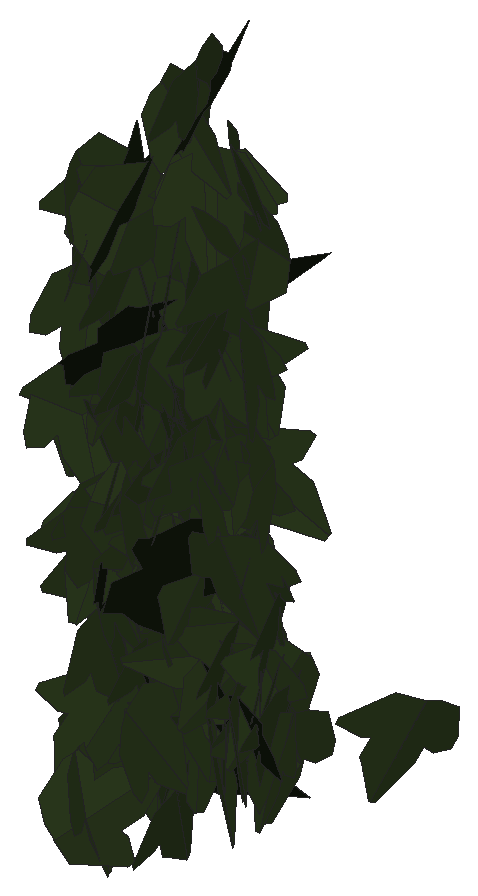
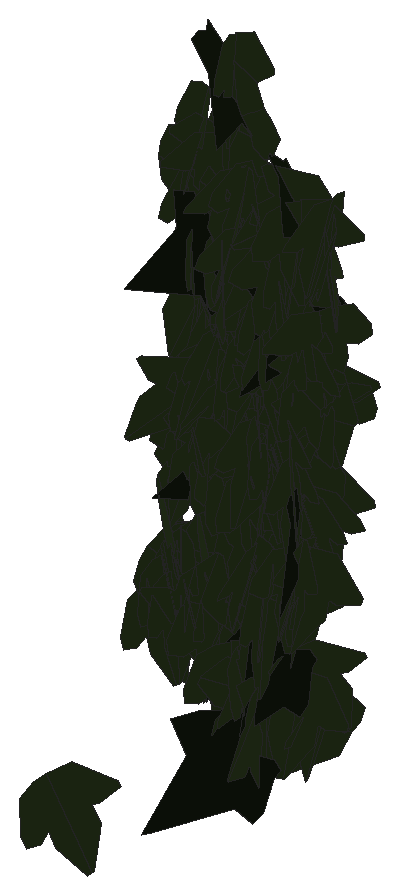
# SketchUp Ruby script. Lengths in inches.
U = 1.inch
M = Sketchup.active_model
def pt(a) = Geom::Point3d.new(a.map { |v| v * U })
def face(e, loops, mat)
  f = e.add_face(loops[0].map { |a| pt(a) })
  loops[1..].each { |l| e.add_face(l.map { |a| pt(a) }).erase! }
  f.material = f.back_material = mat if mat
  f
end
# faces: each face lists its corners as indices into pts; further lists are holes
def faces(e, pts, list, mat = nil) = list.each { |f| face(e, (f[0].is_a?(Array) ? f : [f]).map { |l| l.map { |i| pts[i] } }, mat) }
# xy, xz, yz: faces in a plane at the given z, y or x. An outline is a flat list of corners, or four numbers for a rectangle; further outlines are holes
def ring(l) = l.size == 4 ? [[l[0], l[1]], [l[2], l[1]], [l[2], l[3]], [l[0], l[3]]] : l.each_slice(2).to_a
def flat(e, list, mat, &to3) = list.each { |f| face(e, (f[0].is_a?(Array) ? f : [f]).map { |l| ring(l).map { |u, v| to3.(u, v) } }, mat) }
def xy(e, z, list, mat = nil) = flat(e, list, mat) { |x, y| [x, y, z] }
def xz(e, y, list, mat = nil) = flat(e, list, mat) { |x, z| [x, y, z] }
def yz(e, x, list, mat = nil) = flat(e, list, mat) { |y, z| [x, y, z] }
def lines(e, pts, list) = list.each { |a, b| e.add_line(pt(pts[a]), pt(pts[b])) }
# prism: a flat outline (further loops are holes) pulled along v
def prism(e, loops, v, mat = nil)
  f = face(e, loops, mat); d = Geom::Vector3d.new(v.map { |x| x * U })
  f.pushpull(f.normal.samedirection?(d) ? d.length : -d.length)
end
def box(e, o, s, mat = nil) = prism(e, [[o, [o[0] + s[0], o[1], o[2]], [o[0] + s[0], o[1] + s[1], o[2]], [o[0], o[1] + s[1], o[2]]]], [0, 0, s[2]], mat)
def at(x, y, z, deg = 0) = Geom::Transformation.translation(pt([x, y, z])) * Geom::Transformation.rotation(ORIGIN, Z_AXIS, deg.degrees)
def axes(o, x, y, z) = Geom::Transformation.new([*x, 0, *y, 0, *z, 0, *pt(o).to_a, 1])
def part(name) = M.definitions.add(name)
# library, detail: a bought-in or finely detailed component or shape, given as its bounding box
def library(name, o, s) = part(name).tap { |d| box(d.entities, o, s) }
def detail(e, o, s) = box(e.add_group.entities, o, s)
def put(e, d, t, mat = nil) = e.add_instance(d, t).tap { |i| i.material = mat if mat }
def group(e, t, mat = nil) = e.add_group.tap { |g| g.transformation = t; g.material = mat if mat }.entities
root = M.entities
M.materials.add("efeu1").color = [18, 25, 13]
M.materials.add("efeu2").color = [43, 57, 29]
c1 = part("ivyleaf_10")
p = [[0,0.5,-0.03],[-0.0625,2.02,-0.43],[-0.19,2.01,-0.46],[-0.54,1.05,-0.29],[-0.52,0.625,-0.18],[-0.83,0.76,-0.28],
  [-1.16,0.64,-0.33],[-1.15,0.33,-0.24],[-0.77,-0.39,0.02],[-0.3,-0.51,0.16],[0.04,-0.48,0.23],[-0.02,2.01,-0.4375],
  [-0.06,2.01,-0.43],[0.04,-0.49,0.23],[0.67,-0.49,0.14],[1.38,0.36,-0.2],[1.375,0.51,-0.24],[0.81,0.65,-0.19],
  [0.62,0.59,-0.15],[0.6,1.09,-0.28],[0.5,1.23,-0.31]]
faces(c1.entities,p,[[0,1,2,3,4,5,6,7,8,9,10],[11,12,0,13,14,15,16,17,18,19,20]],"efeu2")
c2 = part("ivyleaf_9")
p = [[1.54,2.16,1.25],[1.36,2.04,1.19],[-0.21,0.99,0.68],[-0.71,1.11,0.82],[-0.85,0.86,0.67],[-0.8,0.17,0.21],
  [-0.9,-0.01,0.1],[-0.67,-0.16,-0.02],[-0.08,-0.08,-0.05],[-0.03,-0.6,-0.4],[0.65,-0.88,-0.66],[0.83,-0.6,-0.49],
  [1.29,-0.42,-0.43],[1.8125,-0.07,-0.26],[1.21,0.44,0.15]]
faces(c2.entities,p,[[0,1,2,3,4,5,6,7,8,9,10,11,12,13,14]],"efeu1")
put(root,c1,axes([23.99,224.85,217.24],[-0.34019,-0.36493,0.03304],[-0.02058,-0.02599,-0.4989],[0.36585,-0.3408,0.00267]))
put(root,c1,axes([24.64,224.9,217.89],[0.32368,-0.38078,-0.01547],[-0.00946,0.01226,-0.49976],[0.38097,0.32382,0.00073]))
put(root,c1,axes([25.13,225,217.29],[-0.20009,-0.41839,0.18685],[-0.0509,-0.18234,-0.46278],[0.45538,-0.20422,0.03038]))
put(root,c2,axes([24.28,224.47,219.45],[0.22776,0.40193,0.19125],[0.09621,0.1653,-0.46197],[-0.43459,0.24724,-0.00205]))
put(root,c2,axes([24.83,224.47,217.24],[0.03415,0.18806,-0.46202],[0.04106,0.46047,0.19047],[0.49714,-0.05095,0.01601]))
put(root,c1,axes([24.84,224.74,220.84],[-0.21282,-0.39948,-0.21243],[0.14447,0.16247,-0.45026],[0.42876,-0.25302,0.04627]))
put(root,c1,axes([24.75,224.9,220.51],[0.32616,-0.37892,-0.00611],[0.04089,0.04321,-0.49645],[0.37676,0.32335,0.05917]))
put(root,c1,axes([25.1,224.79,222.42],[0.03132,-0.47461,-0.15416],[0.0349,0.15617,-0.4737],[0.4978,0.01891,0.04291]))
put(root,c1,axes([25.62,224.77,220.53],[-0.16737,-0.44011,-0.16819],[0.08255,0.14833,-0.4703],[0.46387,-0.1852,0.023]))
put(root,c2,axes([24.43,224.53,220.75],[-0.30098,0.20376,-0.34336],[-0.29499,0.17627,0.36319],[0.26905,0.4212,0.01411]))
put(root,c1,axes([25.23,224.9375,219.86],[0.09069,-0.49135,0.01864],[0.00331,-0.01834,-0.49965],[0.49169,0.09075,-0.00007]))
put(root,c1,axes([23.79,225.01,218.66],[-0.24185,-0.41248,0.14618],[0.00106,-0.16757,-0.47108],[0.43762,-0.22755,0.08192]))
put(root,c1,axes([25.6875,224.71,215.75],[-0.2413,0.39602,0.18692],[-0.17375,0.10933,-0.45592],[-0.40197,-0.28498,0.08485]))
put(root,c1,axes([24.73,224.92,221.91],[0.25831,-0.02532,0.42736],[0.4281,0.01859,-0.25766],[-0.00285,0.49901,0.03128]))
put(root,c1,axes([24.15,224.64,220.76],[0.17757,0.15162,0.44213],[0.27058,0.35231,-0.22948],[-0.38113,0.32076,0.04307]))
put(root,c1,axes([25.53,224.82,217.49],[-0.48309,-0.09874,-0.0829],[0.07973,0.02384,-0.49303],[0.10132,-0.48957,-0.00729]))
put(root,c1,axes([25.24,224.91,221.36],[0.48633,0.09141,0.0716],[0.06671,0.03243,-0.49447],[-0.09504,0.4905,0.01935]))
put(root,c1,axes([25.42,224.9375,219.88],[0.08989,-0.49153,-0.01798],[0.00159,0.01857,-0.49965],[0.49185,0.08977,0.0049]))
put(root,c1,axes([25.03,224.92,218.4375],[0.04642,-0.49708,-0.02748],[0.07532,0.03429,-0.4931],[0.49211,0.04164,0.07806]))
put(root,c1,axes([23.85,224.75,220.44],[0.18326,-0.33537,-0.32241],[-0.16047,0.27968,-0.38213],[0.43665,0.24353,-0.00512]))
put(root,c1,axes([23.68,224.84,218.54],[0.3035,0.38621,0.09343],[0.06226,0.06989,-0.49116],[-0.39244,0.30977,-0.00567]))
put(root,c1,axes([24.48,224.75,217.78],[-0.12293,0.46674,0.13055],[-0.06353,0.11801,-0.4817],[-0.48047,-0.13502,0.03029]))
put(root,c1,axes([23.99,224.97,219.09],[0.45397,-0.20954,0.00105],[0.00697,0.0126,-0.49979],[0.20943,0.4538,0.01436]))
put(root,c1,axes([23.84,224.64,214.15],[0.18589,0.13394,-0.44442],[0.34301,0.28289,0.22873],[0.31271,-0.38991,0.01329]))
put(root,c1,axes([23.91,224.96,217.16],[0.4928,0.03918,-0.07494],[-0.0751,-0.00099,-0.49433],[-0.03888,0.49846,0.00491]))
put(root,c1,axes([25.16,224.84,220.83],[-0.47845,0.14389,0.01949],[-0.02044,-0.00029,-0.49958],[-0.14376,-0.47885,0.00616]))
put(root,c1,axes([24.44,224.91,219.73],[0.3155,-0.37762,-0.08866],[-0.00946,0.10676,-0.48838],[0.38778,0.30984,0.06022]))
put(root,c1,axes([23.66,224.96,220.57],[-0.22607,0.41321,-0.16779],[0.05953,-0.15848,-0.47047],[-0.44198,-0.23269,0.02246]))
put(root,c1,axes([24.375,224.96,219.07],[0.05335,-0.49654,-0.02451],[0.01075,0.0258,-0.49922],[0.49703,0.05274,0.01343]))
put(root,c1,axes([23.98,224.88,218.29],[-0.46009,0.15929,-0.11377],[0.1063,-0.0407,-0.48687],[-0.16437,-0.4722,0.00359]))
put(root,c1,axes([24.59,224.67,215.38],[-0.0733,0.4047,0.28433],[-0.07187,0.27567,-0.4109],[-0.48935,-0.10111,0.01776]))
put(root,c1,axes([24.56,224.8125,219.23],[-0.39362,-0.18683,-0.24527],[0.21446,0.11986,-0.43548],[0.22151,-0.44803,-0.01423]))
put(root,c1,axes([25.2,224.93,221.3],[0.31966,0.38447,0.00162],[0.00126,0.00106,-0.5],[-0.38447,0.31966,-0.00029]))
put(root,c1,axes([25.29,224.83,218.32],[-0.29314,-0.34981,-0.2042],[0.14516,0.1446,-0.45609],[0.37815,-0.32668,0.01678]))
put(root,c1,axes([25.4,224.98,219.99],[0.03875,-0.49697,-0.039],[0.00444,0.03946,-0.49842],[0.49848,0.03828,0.00747]))
put(root,c1,axes([25.03,224.86,220.87],[0.09655,0.48813,0.04903],[-0.01372,0.05264,-0.49703],[-0.4904,0.09463,0.02355]))
put(root,c1,axes([25.23,225.03,218.2],[-0.33588,-0.36203,0.07822],[-0.01051,-0.09624,-0.49054],[0.37024,-0.33116,0.05704]))
put(root,c1,axes([24.25,224.91,220.04],[-0.00537,-0.48085,-0.13693],[0.02096,0.1366,-0.48052],[0.49953,-0.0109,0.01869]))
put(root,c1,axes([23.79,224.88,214.54],[-0.08832,0.49163,0.0224],[-0.0071,0.02149,-0.49949],[-0.49209,-0.08855,0.00319]))
put(root,c1,axes([24,225.02,220.76],[-0.35089,-0.35494,0.02992],[0.04145,-0.0824,-0.49142],[0.35378,-0.34238,0.08725]))
put(root,c1,axes([25.59,224.95,219.73],[-0.41312,0.28161,-0.00477],[-0.04789,-0.07857,-0.49146],[-0.27755,-0.40561,0.09189]))
put(root,c1,axes([24.77,225.13,217.19],[-0.27447,-0.3577,0.21615],[-0.09515,-0.19833,-0.44901],[0.40696,-0.28761,0.0408]))
put(root,c1,axes([23.83,225.21,215.15],[-0.3116,-0.27517,0.27783],[-0.07913,-0.30353,-0.38937],[0.38294,-0.28663,0.14561]))
put(root,c1,axes([24.19,224.82,217.54],[-0.12963,-0.10137,-0.47214],[0.44756,0.15837,-0.15688],[0.18136,-0.46329,0.04968]))
put(root,c1,axes([25.25,225.17,216.19],[0.06994,0.05366,-0.49217],[-0.46028,-0.17601,-0.0846],[-0.18234,0.46491,0.02478]))
put(root,c1,axes([25.6,224.87,221.63],[-0.37901,0.31144,0.09673],[-0.07711,0.05851,-0.49054],[-0.31687,-0.38675,0.00368]))
put(root,c1,axes([23.78,224.875,220.86],[-0.05947,0.48883,0.08667],[-0.04661,0.08141,-0.49112],[-0.49426,-0.0665,0.03588]))
put(root,c1,axes([25.78,224.92,218.4],[0.33466,-0.24246,-0.28145],[-0.19495,0.20784,-0.41085],[0.31622,0.38473,0.04458]))
put(root,c1,axes([24.86,224.86,218.54],[-0.30015,0.27342,0.29181],[-0.28962,0.10296,-0.39436],[-0.27574,-0.40576,0.09657]))
put(root,c1,axes([25.91,224.88,220.82],[0.0117,-0.01087,-0.49975],[-0.43817,0.24035,-0.01548],[0.24056,0.43831,-0.0039]))
put(root,c1,axes([23.87,225.06,217.18],[0.4536,-0.18933,-0.09166],[-0.07809,0.05074,-0.49125],[0.19532,0.45998,0.01646]))
put(root,c1,axes([23.7,225.02,219.55],[0.30312,0.39469,-0.0484],[-0.06469,-0.01111,-0.49567],[-0.39235,0.30676,0.04433]))
put(root,c1,axes([24.45,225.12,217.91],[0.08855,-0.49043,0.04051],[0.01463,-0.03852,-0.4983],[0.49188,0.08943,0.00753]))
put(root,c1,axes([25.27,225,219.57],[-0.47348,0.00141,-0.16066],[0.16008,-0.03869,-0.4721],[-0.01376,-0.4985,0.03618]))
put(root,c1,axes([24.57,224.93,219.29],[-0.03757,-0.46016,-0.19195],[0.00138,0.1924,-0.4615],[0.49858,-0.03521,-0.01319]))
put(root,c1,axes([23.9,225.02,218.77],[-0.40784,-0.22643,-0.17999],[0.20692,-0.01099,-0.45504],[0.20212,-0.44565,0.10267]))
put(root,c1,axes([24.21,225.01,220.11],[-0.44334,-0.20324,-0.1102],[0.12218,-0.00364,-0.48483],[0.19627,-0.45681,0.0529]))
put(root,c1,axes([24.13,225.12,217.75],[0.43914,-0.23761,0.02642],[0.02624,-0.00702,-0.49926],[0.23763,0.43988,0.0063]))
put(root,c1,axes([25.07,224.8125,220.39],[0.20783,-0.30336,-0.33879],[-0.01229,0.36861,-0.3376],[0.4546,0.14865,0.14576]))
put(root,c1,axes([24.74,225,220.16],[-0.29315,-0.36414,-0.17738],[0.2102,0.0504,-0.45086],[0.34624,-0.33891,0.12354]))
put(root,c1,axes([25.4,225.22,216.18],[-0.2869,-0.2613,0.31529],[-0.19686,-0.24957,-0.38596],[0.35908,-0.3456,0.04033]))
put(root,c1,axes([23.84,224.98,216.07],[0.06941,-0.46999,-0.15585],[0.12727,0.16902,-0.45303],[0.47852,0.02321,0.1431]))
put(root,c1,axes([24.86,224.96,218.8],[-0.45899,0.18409,0.07373],[-0.06304,0.04082,-0.49433],[-0.18802,-0.46308,-0.01426]))
put(root,c1,axes([24.78,224.97,218.42],[-0.45079,0.20839,0.05795],[-0.05328,0.02286,-0.49663],[-0.20963,-0.45393,0.00159]))
put(root,c1,axes([25.27,225.11,216.38],[0.18766,-0.46237,-0.03166],[-0.01084,0.02977,-0.499],[0.46332,0.18797,0.00116]))
put(root,c1,axes([24.68,225.05,216.5],[-0.45879,-0.03511,0.19564],[-0.19224,-0.04674,-0.45919],[0.05053,-0.49657,0.02939]))
put(root,c1,axes([24.23,225.07,219.04],[-0.18732,-0.46113,-0.04765],[0.0159,0.04497,-0.49772],[0.46331,-0.18798,-0.00218]))
put(root,c1,axes([24.23,224.93,220.24],[-0.35821,0.3002,0.17766],[-0.15359,0.0929,-0.46667],[-0.3132,-0.38891,0.02566]))
put(root,c1,axes([25.14,224.95,218.38],[0.12281,0.00629,0.48464],[-0.47501,0.10094,0.11906],[-0.09634,-0.48967,0.03077]))
put(root,c1,axes([25.45,224.87,219.5],[0.30335,0.31841,0.23789],[0.03275,0.27822,-0.41415],[-0.39611,0.26685,0.14794]))
put(root,c1,axes([24.24,225.05,219.45],[-0.4916,-0.05956,0.06916],[-0.06766,-0.01645,-0.49513],[0.06126,-0.49617,0.00811]))
put(root,c1,axes([24.2,224.99,219.07],[0.37844,-0.29397,-0.14271],[0.00826,0.22689,-0.44548],[0.32668,0.33482,0.17658]))
put(root,c1,axes([23.92,225.06,217.55],[-0.12643,-0.47058,-0.1121],[0.08585,0.0922,-0.48387],[0.47607,-0.1416,0.05748]))
put(root,c1,axes([25.69,225.41,216.02],[-0.11711,-0.3279,0.35884],[0.04584,-0.37491,-0.32763],[0.48393,-0.04383,0.11787]))
put(root,c1,axes([25.33,225.04,218.27],[0.19107,-0.00989,-0.46194],[-0.44151,0.1435,-0.18569],[0.13625,0.47886,0.04611]))
put(root,c1,axes([25.24,225.01,218.1],[-0.089,0.48941,0.0506],[0.00175,0.05174,-0.49731],[-0.49201,-0.08835,-0.01092]))
put(root,c2,axes([25.26,224.75,222.15],[-0.04942,0.3404,0.36289],[-0.05068,0.35933,-0.34396],[-0.49496,-0.07078,-0.00102]))
put(root,c1,axes([25.29,225.0625,218.09],[-0.48961,-0.06311,-0.07939],[0.07845,0.01239,-0.49365],[0.06427,-0.49585,-0.00223]))
put(root,c1,axes([24.51,225.14,217.18],[-0.24876,-0.43372,0.00228],[-0.00739,0.00161,-0.49994],[0.43366,-0.24876,-0.00721]))
put(root,c1,axes([24.3125,225.14,217.73],[-0.01062,-0.49648,-0.05828],[-0.00686,0.05843,-0.49653],[0.49984,-0.00975,-0.00805]))
put(root,c1,axes([25.49,225.14,217.61],[0.31241,-0.38002,-0.08934],[-0.03704,0.08506,-0.49132],[0.38862,0.3136,0.025]))
put(root,c2,axes([25.31,225,215.8],[0.32476,0.08243,-0.37113],[-0.36571,-0.0656,-0.33459],[-0.10385,0.48878,0.01768]))
put(root,c1,axes([24.2,225.2,218.14],[0.42926,-0.24326,-0.081],[-0.06124,0.05611,-0.49305],[0.24897,0.43322,0.01838]))
put(root,c1,axes([23.99,225.13,217.81],[0.20153,-0.43808,-0.13217],[0.00157,0.14508,-0.47849],[0.45758,0.19245,0.05986]))
put(root,c1,axes([24.5,225.1,217.8],[-0.19392,-0.42304,-0.18285],[0.11229,0.14903,-0.46388],[0.44697,-0.22097,0.03721]))
put(root,c1,axes([25.38,225.15,216.14],[-0.4921,-0.06302,-0.06218],[0.06411,-0.01145,-0.49574],[0.06106,-0.49588,0.01935]))
put(root,c1,axes([24.48,225.15,218.55],[0.47808,0.01489,-0.14567],[-0.14436,0.13124,-0.46036],[0.02452,0.48224,0.12979]))
put(root,c1,axes([25.22,224.99,219.71],[-0.14131,0.08048,0.47282],[-0.39128,0.26572,-0.16217],[-0.27737,-0.41583,-0.01212]))
put(root,c1,axes([25.03,225.24,215.18],[-0.21225,0.44417,-0.08753],[0.02798,-0.08361,-0.49216],[-0.45185,-0.21382,0.01063]))
put(root,c1,axes([24.34,225.28,217.49],[-0.31663,0.36112,-0.13907],[0.04717,-0.14233,-0.47699],[-0.38409,-0.31517,0.05607]))
put(root,c1,axes([25.68,225.34,216.8],[0.21367,-0.45166,0.01856],[0.02416,-0.00909,-0.49933],[0.4514,0.21428,0.01794]))
put(root,c1,axes([25.46,225.1875,217.35],[-0.43957,0.23563,-0.03544],[0.03825,-0.00363,-0.49852],[-0.23519,-0.44098,-0.01483]))
put(root,c1,axes([25.21,225.17,215.47],[-0.221,0.4189,0.16025],[-0.21548,0.05752,-0.44751],[-0.39336,-0.26686,0.15511]))
put(root,c1,axes([25.73,225.38,215.43],[-0.23033,-0.43552,0.08529],[-0.01156,-0.09017,-0.49167],[0.44364,-0.22846,0.03147]))
put(root,c1,axes([25.18,225.14,218.71],[0.01402,-0.42216,-0.26755],[0.12769,0.2618,-0.40639],[0.48322,-0.05693,0.11515]))
put(root,c2,axes([23.98,224.98,217.01],[-0.01586,0.05393,-0.49683],[-0.41834,0.2705,0.04272],[0.27339,0.41704,0.03654]))
put(root,c1,axes([25.7,225.39,215.74],[0.11006,-0.48699,0.02691],[0.00918,-0.02552,-0.49926],[0.48765,0.11039,0.00333]))
put(root,c1,axes([23.73,225.29,216.5],[-0.42364,-0.25908,-0.05839],[0.07275,-0.00749,-0.49462],[0.25541,-0.42758,0.04404]))
put(root,c2,axes([25.25,224.91,219.95],[0.18028,0.22738,0.40718],[0.21455,0.34717,-0.28886],[-0.41408,0.27888,0.02761]))
put(root,c1,axes([24.98,225.22,217.61],[0.32962,0.17669,0.33186],[0.28402,0.17216,-0.37376],[-0.24634,0.43491,0.01313]))
put(root,c1,axes([24.4,225.32,216.55],[0.44294,-0.10678,0.20592],[0.22495,0.08952,-0.43747],[0.05656,0.48019,0.12734]))
put(root,c1,axes([25.38,225.43,215.9375],[0.31505,-0.38069,0.0763],[0.07941,-0.033,-0.49255],[0.38005,0.32247,0.03967]))
put(root,c1,axes([23.85,225.13,216.56],[-0.13852,0.44397,0.18359],[-0.07071,0.17014,-0.46481],[-0.4752,-0.15473,0.01565]))
put(root,c1,axes([25.54,225.45,215.39],[0.434,-0.23327,0.08503],[0.07429,-0.04139,-0.49272],[0.23691,0.44031,-0.00127]))
put(root,c1,axes([25.55,225.4375,215.85],[-0.12446,-0.47938,0.0686],[-0.01168,-0.06783,-0.49524],[0.48412,-0.12488,0.00569]))
put(root,c1,axes([24.5,225.28,216.4],[-0.13395,0.48159,0.01115],[0.00786,0.01376,-0.49975],[-0.48166,-0.13371,-0.01125]))
put(root,c1,axes([25.41,225.17,218.21],[0.22802,0.22611,0.38325],[0.24416,0.29644,-0.32017],[-0.37201,0.33316,0.02477]))
put(root,c1,axes([24.9,225.42,215.53],[-0.39058,-0.30702,0.05645],[-0.02692,-0.05695,-0.49602],[0.31101,-0.3905,0.02795]))
put(root,c1,axes([23.8125,225.34,214.91],[-0.48386,-0.12506,-0.01531],[0.01253,0.0127,-0.49968],[0.12537,-0.48394,-0.00915]))
put(root,c1,axes([24.48,225.29,214.31],[0.02971,-0.4459,-0.22425],[-0.0011,0.22459,-0.44672],[0.49912,0.02703,0.01236]))
put(root,c1,axes([23.89,225.34,216.63],[-0.45178,0.17177,0.12802],[-0.13441,0.00539,-0.48157],[-0.16682,-0.46954,0.0413]))
put(root,c1,axes([24.22,225.36,215.87],[-0.01184,-0.47475,-0.15644],[0.02032,0.15589,-0.47464],[0.49945,-0.0176,0.0156]))
put(root,c1,axes([25,225.39,215.7],[0.27086,0.02559,0.4195],[0.40235,0.12844,-0.26762],[-0.12146,0.48254,0.04899]))
put(root,c1,axes([24.4,225.52,215.09],[0.08989,-0.49156,0.01712],[0.00301,-0.01686,-0.49971],[0.49184,0.08994,-0.00008]))
put(root,c1,axes([24.11,225.52,214.83],[-0.31428,-0.38841,0.01922],[0.06727,-0.07864,-0.48917],[0.38302,-0.30488,0.10169]))
put(root,c1,axes([24.34,225.29,216.29],[-0.36214,0.24534,0.2422],[-0.20894,0.12321,-0.43722],[-0.27422,-0.41788,0.01329]))
put(root,c1,axes([25.45,225.46,215.66],[-0.03889,-0.49312,-0.07294],[0.00291,0.07294,-0.49464],[0.49848,-0.0389,-0.0028]))
put(root,c1,axes([25.52,225.5,216],[0.26289,-0.42269,-0.04712],[-0.00313,0.05347,-0.49712],[0.4253,0.26167,0.02547]))
put(root,c1,axes([25.35,225.42,216.23],[0.34315,-0.34289,-0.12115],[0.01615,0.18077,-0.4659],[0.3633,0.31583,0.13514]))
put(root,c1,axes([24.59,225.54,215.09],[-0.31871,-0.38453,0.02374],[0.03387,-0.05866,-0.49539],[0.38377,-0.31416,0.06344]))
put(root,c2,axes([23.98,225.34,215.36],[0.48825,0.07948,-0.07278],[-0.07227,-0.00902,-0.49467],[-0.07994,0.49356,0.00268]))
put(root,c1,axes([25.1,225.52,215.55],[0.4015,0.27583,0.11276],[-0.11129,-0.03671,0.48607],[0.27643,-0.41541,0.03192]))
put(root,c1,axes([24.4,225.48,214.78],[0.06072,-0.28175,0.40857],[-0.10789,0.39428,0.28792],[-0.48443,-0.12312,-0.01292]))
put(root,c1,axes([23.96,225.92,214.7],[0.01724,-0.09635,-0.49033],[-0.08599,0.48273,-0.09788],[0.49225,0.0877,0.00008]))
put(root,c2,axes([24.08,225.95,214.28],[0.37092,0.2751,0.19167],[0.15283,0.11568,-0.4618],[-0.29843,0.40117,0.00173]))
put(root,c1,axes([25.18,227.96,214.26],[-0.23113,-0.4029,0.18508],[-0.10256,-0.15447,-0.46435],[0.43135,-0.25261,-0.01124]))
